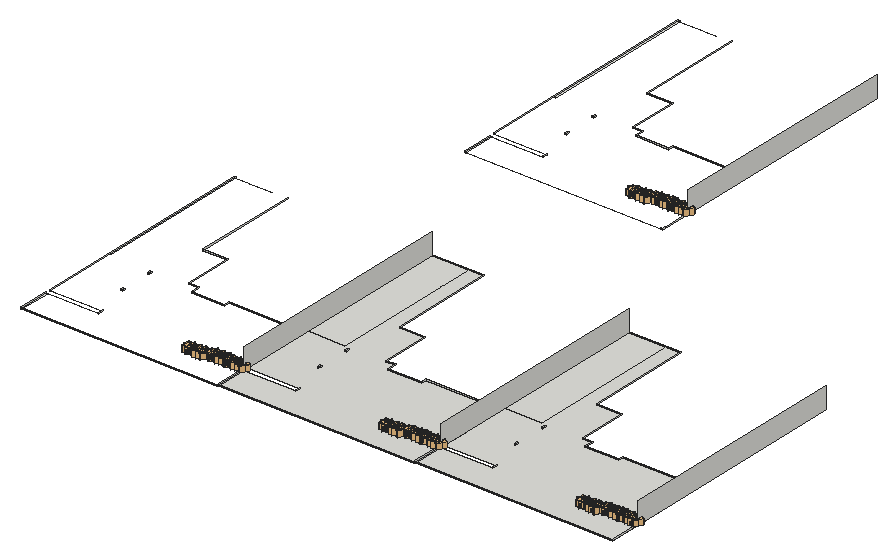
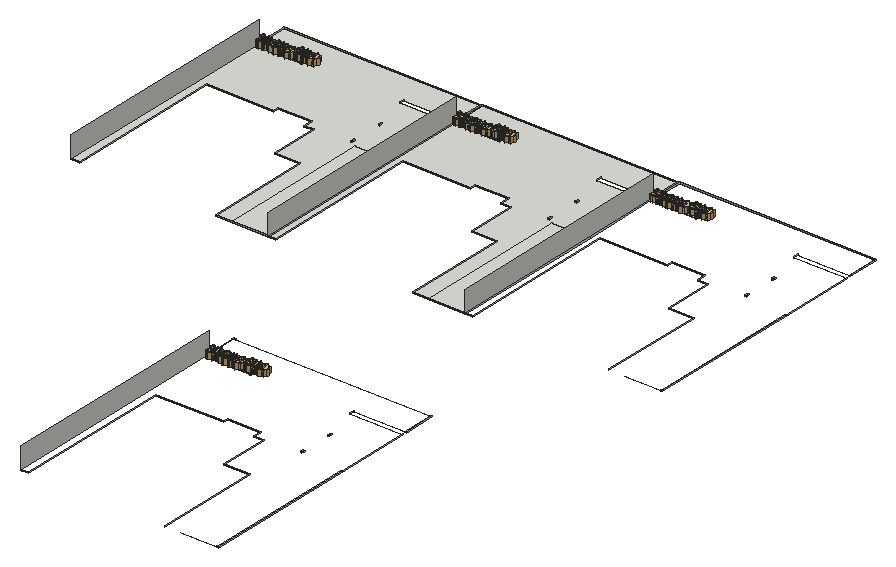
# SketchUp Ruby script. Lengths in inches.
U = 1.inch
M = Sketchup.active_model
def pt(a) = Geom::Point3d.new(a.map { |v| v * U })
def face(e, loops, mat)
  f = e.add_face(loops[0].map { |a| pt(a) })
  loops[1..].each { |l| e.add_face(l.map { |a| pt(a) }).erase! }
  f.material = f.back_material = mat if mat
  f
end
# faces: each face lists its corners as indices into pts; further lists are holes
def faces(e, pts, list, mat = nil) = list.each { |f| face(e, (f[0].is_a?(Array) ? f : [f]).map { |l| l.map { |i| pts[i] } }, mat) }
# xy, xz, yz: faces in a plane at the given z, y or x. An outline is a flat list of corners, or four numbers for a rectangle; further outlines are holes
def ring(l) = l.size == 4 ? [[l[0], l[1]], [l[2], l[1]], [l[2], l[3]], [l[0], l[3]]] : l.each_slice(2).to_a
def flat(e, list, mat, &to3) = list.each { |f| face(e, (f[0].is_a?(Array) ? f : [f]).map { |l| ring(l).map { |u, v| to3.(u, v) } }, mat) }
def xy(e, z, list, mat = nil) = flat(e, list, mat) { |x, y| [x, y, z] }
def xz(e, y, list, mat = nil) = flat(e, list, mat) { |x, z| [x, y, z] }
def yz(e, x, list, mat = nil) = flat(e, list, mat) { |y, z| [x, y, z] }
def lines(e, pts, list) = list.each { |a, b| e.add_line(pt(pts[a]), pt(pts[b])) }
# prism: a flat outline (further loops are holes) pulled along v
def prism(e, loops, v, mat = nil)
  f = face(e, loops, mat); d = Geom::Vector3d.new(v.map { |x| x * U })
  f.pushpull(f.normal.samedirection?(d) ? d.length : -d.length)
end
def box(e, o, s, mat = nil) = prism(e, [[o, [o[0] + s[0], o[1], o[2]], [o[0] + s[0], o[1] + s[1], o[2]], [o[0], o[1] + s[1], o[2]]]], [0, 0, s[2]], mat)
def at(x, y, z, deg = 0) = Geom::Transformation.translation(pt([x, y, z])) * Geom::Transformation.rotation(ORIGIN, Z_AXIS, deg.degrees)
def axes(o, x, y, z) = Geom::Transformation.new([*x, 0, *y, 0, *z, 0, *pt(o).to_a, 1])
def part(name) = M.definitions.add(name)
# library, detail: a bought-in or finely detailed component or shape, given as its bounding box
def library(name, o, s) = part(name).tap { |d| box(d.entities, o, s) }
def detail(e, o, s) = box(e.add_group.entities, o, s)
def put(e, d, t, mat = nil) = e.add_instance(d, t).tap { |i| i.material = mat if mat }
def group(e, t, mat = nil) = e.add_group.tap { |g| g.transformation = t; g.material = mat if mat }.entities
root = M.entities
M.materials.add("[Color_F16]").color = [51, 102, 0]
M.materials.add("[Field Square Tile]").color = [217, 201, 169]
c1 = library("Obj_000003",[-31,-31.06,-7.89],[62,62.12,39.58])
xy(root,-23.875,[[68.91,0,75.99,143.39],[955.37,0,962.46,143.39],[[962.46,0,962.46,143.39,1194.85,143.39,1194.85,164.82,962.46,164.82,962.46,505.3125,1127.79,505.3125,1127.79,1201.875,1196.48,1201.875,1196.48,726.125,1310.86,726.125,1310.86,505.3125,1354.48,505.3125,1354.48,464.0625,1504.89,464.0625,1504.89,487.3125,1810.23,487.3125,1810.23,1201.875,1841.83,1201.875,1841.83,164.82,1848.92,164.82,1848.92,143.39,1841.83,143.39,1841.83,0],[1150.61,475.3125,1157.34,487.3125],[1150.61,322.71,1157.34,334.4375]],[1841.83,0,1848.92,143.39],[[1848.92,0,1848.92,143.39,2081.32,143.39,2081.32,164.82,1848.92,164.82,1848.92,505.3125,2014.26,505.3125,2014.26,1201.875,2082.95,1201.875,2082.95,726.125,2197.32,726.125,2197.32,505.3125,2240.94,505.3125,2240.94,464.0625,2391.36,464.0625,2391.36,487.3125,2696.7,487.3125,2696.7,1201.875,2735.38,1201.875,2735.38,0],[2037.07,475.3125,2043.8,487.3125],[2037.07,322.71,2043.8,334.4375]],
  [955.37,164.82,962.46,505.3125],[1841.83,164.82,1848.92,505.3125],[68.91,505.3125,75.99,1201.875],[955.37,505.3125,962.46,1201.875],[962.46,505.3125,1127.79,1201.875],
  [1841.83,505.3125,1848.92,1201.875],[1848.92,505.3125,2014.26,1201.875],[587.64,1851.99,594.72,1995.38],[587.64,2357.31,594.72,3053.87]])
xy(root,-20.8125,[[747.55,143.39,901.18,164.82],[1634.02,143.39,1787.65,164.82],[2520.48,143.39,2674.11,164.82],[1266.28,1995.38,1419.92,2016.82]])
xz(root,0,[[75.99,-23.875,955.37,-19.3125],[955.37,-23.875,962.46,-19.3125],[962.46,-23.875,1841.83,-19.3125],[1841.83,-23.875,1848.92,-19.3125],[1848.92,-23.875,2735.38,-19.3125]],"[Field Square Tile]")
xz(root,143.39,[[747.55,-20.8125,901.18,-19.75],[1634.02,-20.8125,1787.65,-19.75],[2520.48,-20.8125,2674.11,-19.75]])
xz(root,164.82,[[747.55,-20.8125,901.18,-19.75],[1634.02,-20.8125,1787.65,-19.75],[2520.48,-20.8125,2674.11,-19.75]])
xz(root,322.71,[[264.14,-23.875,270.875,-19.75],[1150.61,-23.875,1157.34,-19.75],[2037.07,-23.875,2043.8,-19.75]])
xz(root,334.4375,[[264.14,-23.875,270.875,-19.75],[1150.61,-23.875,1157.34,-19.75],[2037.07,-23.875,2043.8,-19.75]])
xz(root,464.0625,[[468.02,-23.875,618.43,-19.75],[1354.48,-23.875,1504.89,-19.75],[2240.94,-23.875,2391.36,-19.75]])
xz(root,475.3125,[[264.14,-23.875,270.875,-19.75],[1150.61,-23.875,1157.34,-19.75],[2037.07,-23.875,2043.8,-19.75]])
xz(root,487.3125,[[264.14,-23.875,270.875,-19.75],[618.43,-23.875,923.77,-19.75],[1150.61,-23.875,1157.34,-19.75],[1504.89,-23.875,1810.23,-19.75],[2037.07,-23.875,2043.8,-19.75],
  [2391.36,-23.875,2696.7,-19.75]])
xz(root,505.3125,[[424.39,-23.875,468.02,-19.75],[1310.86,-23.875,1354.48,-19.75],[2197.32,-23.875,2240.94,-19.75]])
xz(root,726.125,[[310.02,-23.875,424.39,-19.75],[1196.48,-23.875,1310.86,-19.75],[2082.95,-23.875,2197.32,-19.75]])
xz(root,1201.875,[[68.91,-23.875,75.99,-19.75],[923.77,-23.875,955.37,-19.75],[955.37,-23.875,962.46,-19.75],[962.46,-23.875,1196.48,-19.75],[1810.23,-23.875,1841.83,-19.75],
  [1841.83,-23.875,1848.92,-19.75],[1848.92,-23.875,2082.95,-19.75],[2696.7,-23.875,2735.38,-19.75]])
xz(root,1851.99,[[1474.1,-23.875,1481.1875,-19.3125]],"[Field Square Tile]")
xz(root,1995.38,[[1266.28,-20.8125,1419.92,-19.75]])
xz(root,2016.82,[[1266.28,-20.8125,1419.92,-19.75]])
xz(root,2174.7,[[782.875,-23.875,789.61,-19.75]])
xz(root,2186.43,[[782.875,-23.875,789.61,-19.75]])
xz(root,2316.06,[[986.75,-23.875,1137.16,-19.75]])
xz(root,2327.31,[[782.875,-23.875,789.61,-19.75]])
xz(root,2339.31,[[782.875,-23.875,789.61,-19.75],[1137.16,-23.875,1442.5,-19.75]])
xz(root,2357.31,[[943.125,-23.875,986.75,-19.75]])
xz(root,2578.12,[[828.75,-23.875,943.125,-19.75]])
xz(root,3053.87,[[587.64,-23.875,594.72,-19.75],[1442.5,-23.875,1474.1,-19.75]])
yz(root,68.91,[[0,-23.875,0,-19.3125,12.39,-19.3125,12.39,-19.75,143.39,-19.75,143.39,-23.875],[164.82,-23.875,505.3125,-19.75],[505.3125,-23.875,1201.875,-19.75]])
yz(root,264.14,[[322.71,-23.875,334.4375,-19.75],[475.3125,-23.875,487.3125,-19.75]])
yz(root,270.875,[[322.71,-23.875,334.4375,-19.75],[475.3125,-23.875,487.3125,-19.75]])
yz(root,308.39,[[143.39,-23.875,164.82,-19.75]])
yz(root,310.02,[[726.125,-23.875,1201.875,-19.75]])
yz(root,424.39,[[505.3125,-23.875,726.125,-19.75]])
yz(root,468.02,[[464.0625,-23.875,505.3125,-19.75]])
yz(root,587.64,[[1851.99,-23.875,1851.99,-19.3125,1864.38,-19.3125,1864.38,-19.75,1995.38,-19.75,1995.38,-23.875],[2016.82,-23.875,2357.31,-19.75],[2357.31,-23.875,3053.87,-19.75]])
yz(root,618.43,[[464.0625,-23.875,487.3125,-19.75]])
yz(root,782.875,[[2174.7,-23.875,2186.43,-19.75],[2327.31,-23.875,2339.31,-19.75]])
yz(root,789.61,[[2174.7,-23.875,2186.43,-19.75],[2327.31,-23.875,2339.31,-19.75]])
yz(root,827.12,[[1995.38,-23.875,2016.82,-19.75]])
yz(root,828.75,[[2578.12,-23.875,3053.87,-19.75]])
yz(root,923.77,[[487.3125,-23.875,1201.875,-19.75]])
yz(root,943.125,[[2357.31,-23.875,2578.12,-19.75]])
yz(root,955.37,[[0,-23.875,0,-19.3125,12.39,-19.3125,12.39,-19.75,143.39,-19.75,143.39,-23.875],[164.82,-23.875,505.3125,-19.75],[505.3125,-23.875,1201.875,-19.75]])
yz(root,962.46,[[0,-23.875,1201.875,-23.875,1201.875,73,143.39,73,143.39,-19.75,12.39,-19.75,12.39,-19.3125,0,-19.3125]])
yz(root,986.75,[[2316.06,-23.875,2357.31,-19.75]])
yz(root,1137.16,[[2316.06,-23.875,2339.31,-19.75]])
yz(root,1150.61,[[322.71,-23.875,334.4375,-19.75],[475.3125,-23.875,487.3125,-19.75]])
yz(root,1157.34,[[322.71,-23.875,334.4375,-19.75],[475.3125,-23.875,487.3125,-19.75]])
yz(root,1194.85,[[143.39,-23.875,164.82,-19.75]])
yz(root,1196.48,[[726.125,-23.875,1201.875,-19.75]])
yz(root,1310.86,[[505.3125,-23.875,726.125,-19.75]])
yz(root,1354.48,[[464.0625,-23.875,505.3125,-19.75]])
yz(root,1442.5,[[2339.31,-23.875,3053.87,-19.75]])
yz(root,1481.1875,[[1851.99,-23.875,3053.87,-23.875,3053.87,73,1995.38,73,1995.38,-19.75,1864.38,-19.75,1864.38,-19.3125,1851.99,-19.3125]])
yz(root,1504.89,[[464.0625,-23.875,487.3125,-19.75]])
yz(root,1810.23,[[487.3125,-23.875,1201.875,-19.75]])
yz(root,1841.83,[[0,-23.875,0,-19.3125,12.39,-19.3125,12.39,-19.75,143.39,-19.75,143.39,-23.875],[164.82,-23.875,505.3125,-19.75],[505.3125,-23.875,1201.875,-19.75]])
yz(root,1848.92,[[0,-23.875,1201.875,-23.875,1201.875,73,143.39,73,143.39,-19.75,12.39,-19.75,12.39,-19.3125,0,-19.3125]])
yz(root,2037.07,[[322.71,-23.875,334.4375,-19.75],[475.3125,-23.875,487.3125,-19.75]])
yz(root,2043.8,[[322.71,-23.875,334.4375,-19.75],[475.3125,-23.875,487.3125,-19.75]])
yz(root,2081.32,[[143.39,-23.875,164.82,-19.75]])
yz(root,2082.95,[[726.125,-23.875,1201.875,-19.75]])
yz(root,2197.32,[[505.3125,-23.875,726.125,-19.75]])
yz(root,2240.94,[[464.0625,-23.875,505.3125,-19.75]])
yz(root,2391.36,[[464.0625,-23.875,487.3125,-19.75]])
yz(root,2696.7,[[487.3125,-23.875,1201.875,-19.75]])
yz(root,2735.38,[[0,-23.875,1201.875,-23.875,1201.875,73,143.39,73,143.39,-19.75,12.39,-19.75,12.39,-19.3125,0,-19.3125]])
p = [[308.39,164.82,-23.875],[75.99,164.82,-23.875],[241.33,1201.875,-23.875],[75.99,1201.875,-23.875],[75.99,143.39,-23.875],[308.39,143.39,-23.875],
  [68.91,164.82,-23.875],[594.72,1851.99,-19.3125],[594.72,1851.99,-23.875],[760.06,3053.87,-23.875],[594.72,3053.87,-23.875],[827.12,2016.82,-23.875],
  [594.72,2016.82,-23.875],[594.72,1995.38,-23.875],[827.12,1995.38,-23.875],[587.64,2016.82,-23.875],[1474.1,1851.99,-23.875]]
lines(root,p,[[0,1],[2,3],[4,5],[1,6],[7,8],[9,10],[11,12],[13,14],[12,15],[8,16]])
put(root,c1,axes([1630.48,130.4,-17.02],[-0.16941,0.61717,-0.00035],[-0.61717,-0.16941,0.00015],[0.00005,0.00038,0.64]),"[Color_F16]")
put(root,c1,axes([1662.26,130.18,-17.02],[0.45255,0.45255,-0.00035],[-0.45255,0.45255,0.00015],[0.00035,0.00015,0.64]),"[Color_F16]")
put(root,c1,axes([1646.38,130.18,-17.02],[0.45255,0.45255,-0.00035],[-0.45255,0.45255,0.00015],[0.00035,0.00015,0.64]),"[Color_F16]")
put(root,c1,axes([1614.64,130.18,-17.02],[0.45255,0.45255,-0.00035],[-0.45255,0.45255,0.00015],[0.00035,0.00015,0.64]),"[Color_F16]")
put(root,c1,axes([1676.95,129.48,-17.02],[0.34155,0.54124,-0.00035],[-0.54124,0.34155,0.00015],[0.00031,0.00022,0.64]),"[Color_F16]")
put(root,c1,axes([2501.1,130.18,-17.02],[0.45255,0.45255,-0.00035],[-0.45255,0.45255,0.00015],[0.00035,0.00015,0.64]),"[Color_F16]")
put(root,c1,axes([2563.41,129.48,-17.02],[0.34155,0.54124,-0.00035],[-0.54124,0.34155,0.00015],[0.00031,0.00022,0.64]),"[Color_F16]")
put(root,c1,axes([2516.95,130.4,-17.02],[-0.16941,0.61717,-0.00035],[-0.61717,-0.16941,0.00015],[0.00005,0.00038,0.64]),"[Color_F16]")
put(root,c1,axes([2548.72,130.18,-17.02],[0.45255,0.45255,-0.00035],[-0.45255,0.45255,0.00015],[0.00035,0.00015,0.64]),"[Color_F16]")
put(root,c1,axes([2532.85,130.18,-17.02],[0.45255,0.45255,-0.00035],[-0.45255,0.45255,0.00015],[0.00035,0.00015,0.64]),"[Color_F16]")
put(root,c1,axes([790.48,129.48,-17.02],[0.34155,0.54124,-0.00035],[-0.54124,0.34155,0.00015],[0.00031,0.00022,0.64]),"[Color_F16]")
put(root,c1,axes([744.02,130.4,-17.02],[-0.16941,0.61717,-0.00035],[-0.61717,-0.16941,0.00015],[0.00005,0.00038,0.64]),"[Color_F16]")
put(root,c1,axes([728.17,130.18,-17.02],[0.45255,0.45255,-0.00035],[-0.45255,0.45255,0.00015],[0.00035,0.00015,0.64]),"[Color_F16]")
put(root,c1,axes([775.79,130.18,-17.02],[0.45255,0.45255,-0.00035],[-0.45255,0.45255,0.00015],[0.00035,0.00015,0.64]),"[Color_F16]")
put(root,c1,axes([759.92,130.18,-17.02],[0.45255,0.45255,-0.00035],[-0.45255,0.45255,0.00015],[0.00035,0.00015,0.64]),"[Color_F16]")
put(root,c1,axes([1278.65,1982.18,-17.02],[0.45255,0.45255,-0.00035],[-0.45255,0.45255,0.00015],[0.00035,0.00015,0.64]),"[Color_F16]")
put(root,c1,axes([1294.53,1982.18,-17.02],[0.45255,0.45255,-0.00035],[-0.45255,0.45255,0.00015],[0.00035,0.00015,0.64]),"[Color_F16]")
put(root,c1,axes([1262.75,1982.39,-17.02],[-0.16941,0.61717,-0.00035],[-0.61717,-0.16941,0.00015],[0.00005,0.00038,0.64]),"[Color_F16]")
put(root,c1,axes([1246.9,1982.18,-17.02],[0.45255,0.45255,-0.00035],[-0.45255,0.45255,0.00015],[0.00035,0.00015,0.64]),"[Color_F16]")
put(root,c1,axes([1309.22,1981.47,-17.02],[0.34155,0.54124,-0.00035],[-0.54124,0.34155,0.00015],[0.00031,0.00022,0.64]),"[Color_F16]")
put(root,c1,axes([1677.44,130.52,-17.02],[0.28256,0.57425,0],[-0.57425,0.28256,0],[0,0,0.64]),"[Color_F16]")
put(root,c1,axes([1614.23,130.26,-17.02],[0.64,0,0],[0,0.64,0],[0,0,0.64]),"[Color_F16]")
put(root,c1,axes([1630.48,130.71,-17.02],[-0.15049,0.62206,0],[-0.62206,-0.15049,0],[0,0,0.64]),"[Color_F16]")
put(root,c1,axes([1645.97,130.26,-17.02],[0.64,0,0],[0,0.64,0],[0,0,0.64]),"[Color_F16]")
put(root,c1,axes([1661.85,130.26,-17.02],[0.64,0,0],[0,0.64,0],[0,0,0.64]),"[Color_F16]")
put(root,c1,axes([2532.4375,130.26,-17.02],[0.64,0,0],[0,0.64,0],[0,0,0.64]),"[Color_F16]")
put(root,c1,axes([2563.9,130.52,-17.02],[0.28256,0.57425,0],[-0.57425,0.28256,0],[0,0,0.64]),"[Color_F16]")
put(root,c1,axes([2500.69,130.26,-17.02],[0.64,0,0],[0,0.64,0],[0,0,0.64]),"[Color_F16]")
put(root,c1,axes([2516.95,130.71,-17.02],[-0.15049,0.62206,0],[-0.62206,-0.15049,0],[0,0,0.64]),"[Color_F16]")
put(root,c1,axes([2548.3125,130.26,-17.02],[0.64,0,0],[0,0.64,0],[0,0,0.64]),"[Color_F16]")
put(root,c1,axes([759.51,130.26,-17.02],[0.64,0,0],[0,0.64,0],[0,0,0.64]),"[Color_F16]")
put(root,c1,axes([727.76,130.26,-17.02],[0.64,0,0],[0,0.64,0],[0,0,0.64]),"[Color_F16]")
put(root,c1,axes([790.97,130.52,-17.02],[0.28256,0.57425,0],[-0.57425,0.28256,0],[0,0,0.64]),"[Color_F16]")
put(root,c1,axes([744.02,130.71,-17.02],[-0.15049,0.62206,0],[-0.62206,-0.15049,0],[0,0,0.64]),"[Color_F16]")
put(root,c1,axes([775.38,130.26,-17.02],[0.64,0,0],[0,0.64,0],[0,0,0.64]),"[Color_F16]")
put(root,c1,axes([1262.75,1982.71,-17.02],[-0.15049,0.62206,0],[-0.62206,-0.15049,0],[0,0,0.64]),"[Color_F16]")
put(root,c1,axes([1309.7,1982.52,-17.02],[0.28256,0.57425,0],[-0.57425,0.28256,0],[0,0,0.64]),"[Color_F16]")
put(root,c1,axes([1278.24,1982.25,-17.02],[0.64,0,0],[0,0.64,0],[0,0,0.64]),"[Color_F16]")
put(root,c1,axes([1246.49,1982.25,-17.02],[0.64,0,0],[0,0.64,0],[0,0,0.64]),"[Color_F16]")
put(root,c1,axes([1294.12,1982.25,-17.02],[0.64,0,0],[0,0.64,0],[0,0,0.64]),"[Color_F16]")
put(root,c1,axes([1708.47,144.13,-16.22],[0.45255,0.45255,-0.00035],[-0.45255,0.45255,0.00015],[0.00035,0.00015,0.64]),"[Color_F16]")
put(root,c1,axes([1770.79,143.43,-16.22],[0.34155,0.54124,-0.00035],[-0.54124,0.34155,0.00015],[0.00031,0.00022,0.64]),"[Color_F16]")
put(root,c1,axes([1724.32,144.35,-16.22],[-0.16941,0.61717,-0.00035],[-0.61717,-0.16941,0.00015],[0.00005,0.00038,0.64]),"[Color_F16]")
put(root,c1,axes([1756.1,144.13,-16.22],[0.45255,0.45255,-0.00035],[-0.45255,0.45255,0.00015],[0.00035,0.00015,0.64]),"[Color_F16]")
put(root,c1,axes([1740.22,144.13,-16.22],[0.45255,0.45255,-0.00035],[-0.45255,0.45255,0.00015],[0.00035,0.00015,0.64]),"[Color_F16]")
put(root,c1,axes([1841.16,143.43,-16.22],[0.34155,0.54124,-0.00035],[-0.54124,0.34155,0.00015],[0.00031,0.00022,0.64]),"[Color_F16]")
put(root,c1,axes([1778.85,144.13,-16.22],[0.45255,0.45255,-0.00035],[-0.45255,0.45255,0.00015],[0.00035,0.00015,0.64]),"[Color_F16]")
put(root,c1,axes([1794.7,144.35,-16.22],[-0.16941,0.61717,-0.00035],[-0.61717,-0.16941,0.00015],[0.00005,0.00038,0.64]),"[Color_F16]")
put(root,c1,axes([1826.47,144.13,-16.22],[0.45255,0.45255,-0.00035],[-0.45255,0.45255,0.00015],[0.00035,0.00015,0.64]),"[Color_F16]")
put(root,c1,axes([1810.6,144.13,-16.22],[0.45255,0.45255,-0.00035],[-0.45255,0.45255,0.00015],[0.00035,0.00015,0.64]),"[Color_F16]")
put(root,c1,axes([2697.06,144.13,-16.22],[0.45255,0.45255,-0.00035],[-0.45255,0.45255,0.00015],[0.00035,0.00015,0.64]),"[Color_F16]")
put(root,c1,axes([2712.93,144.13,-16.22],[0.45255,0.45255,-0.00035],[-0.45255,0.45255,0.00015],[0.00035,0.00015,0.64]),"[Color_F16]")
put(root,c1,axes([2681.16,144.35,-16.22],[-0.16941,0.61717,-0.00035],[-0.61717,-0.16941,0.00015],[0.00005,0.00038,0.64]),"[Color_F16]")
put(root,c1,axes([2665.3125,144.13,-16.22],[0.45255,0.45255,-0.00035],[-0.45255,0.45255,0.00015],[0.00035,0.00015,0.64]),"[Color_F16]")
put(root,c1,axes([2727.625,143.43,-16.22],[0.34155,0.54124,-0.00035],[-0.54124,0.34155,0.00015],[0.00031,0.00022,0.64]),"[Color_F16]")
put(root,c1,axes([2657.25,143.43,-16.22],[0.34155,0.54124,-0.00035],[-0.54124,0.34155,0.00015],[0.00031,0.00022,0.64]),"[Color_F16]")
put(root,c1,axes([2594.9375,144.13,-16.22],[0.45255,0.45255,-0.00035],[-0.45255,0.45255,0.00015],[0.00035,0.00015,0.64]),"[Color_F16]")
put(root,c1,axes([2610.79,144.35,-16.22],[-0.16941,0.61717,-0.00035],[-0.61717,-0.16941,0.00015],[0.00005,0.00038,0.64]),"[Color_F16]")
put(root,c1,axes([2642.56,144.13,-16.22],[0.45255,0.45255,-0.00035],[-0.45255,0.45255,0.00015],[0.00035,0.00015,0.64]),"[Color_F16]")
put(root,c1,axes([2626.69,144.13,-16.22],[0.45255,0.45255,-0.00035],[-0.45255,0.45255,0.00015],[0.00035,0.00015,0.64]),"[Color_F16]")
put(root,c1,axes([892.38,144.13,-16.22],[0.45255,0.45255,-0.00035],[-0.45255,0.45255,0.00015],[0.00035,0.00015,0.64]),"[Color_F16]")
put(root,c1,axes([908.23,144.35,-16.22],[-0.16941,0.61717,-0.00035],[-0.61717,-0.16941,0.00015],[0.00005,0.00038,0.64]),"[Color_F16]")
put(root,c1,axes([924.13,144.13,-16.22],[0.45255,0.45255,-0.00035],[-0.45255,0.45255,0.00015],[0.00035,0.00015,0.64]),"[Color_F16]")
put(root,c1,axes([940.01,144.13,-16.22],[0.45255,0.45255,-0.00035],[-0.45255,0.45255,0.00015],[0.00035,0.00015,0.64]),"[Color_F16]")
put(root,c1,axes([954.7,143.43,-16.22],[0.34155,0.54124,-0.00035],[-0.54124,0.34155,0.00015],[0.00031,0.00022,0.64]),"[Color_F16]")
put(root,c1,axes([884.32,143.43,-16.22],[0.34155,0.54124,-0.00035],[-0.54124,0.34155,0.00015],[0.00031,0.00022,0.64]),"[Color_F16]")
put(root,c1,axes([822.01,144.13,-16.22],[0.45255,0.45255,-0.00035],[-0.45255,0.45255,0.00015],[0.00035,0.00015,0.64]),"[Color_F16]")
put(root,c1,axes([869.63,144.13,-16.22],[0.45255,0.45255,-0.00035],[-0.45255,0.45255,0.00015],[0.00035,0.00015,0.64]),"[Color_F16]")
put(root,c1,axes([837.86,144.35,-16.22],[-0.16941,0.61717,-0.00035],[-0.61717,-0.16941,0.00015],[0.00005,0.00038,0.64]),"[Color_F16]")
put(root,c1,axes([853.76,144.13,-16.22],[0.45255,0.45255,-0.00035],[-0.45255,0.45255,0.00015],[0.00035,0.00015,0.64]),"[Color_F16]")
put(root,c1,axes([1442.86,1996.125,-16.22],[0.45255,0.45255,-0.00035],[-0.45255,0.45255,0.00015],[0.00035,0.00015,0.64]),"[Color_F16]")
put(root,c1,axes([1403.05,1995.42,-16.22],[0.34155,0.54124,-0.00035],[-0.54124,0.34155,0.00015],[0.00031,0.00022,0.64]),"[Color_F16]")
put(root,c1,axes([1340.74,1996.125,-16.22],[0.45255,0.45255,-0.00035],[-0.45255,0.45255,0.00015],[0.00035,0.00015,0.64]),"[Color_F16]")
put(root,c1,axes([1388.36,1996.125,-16.22],[0.45255,0.45255,-0.00035],[-0.45255,0.45255,0.00015],[0.00035,0.00015,0.64]),"[Color_F16]")
put(root,c1,axes([1458.74,1996.125,-16.22],[0.45255,0.45255,-0.00035],[-0.45255,0.45255,0.00015],[0.00035,0.00015,0.64]),"[Color_F16]")
put(root,c1,axes([1411.12,1996.125,-16.22],[0.45255,0.45255,-0.00035],[-0.45255,0.45255,0.00015],[0.00035,0.00015,0.64]),"[Color_F16]")
put(root,c1,axes([1426.96,1996.34,-16.22],[-0.16941,0.61717,-0.00035],[-0.61717,-0.16941,0.00015],[0.00005,0.00038,0.64]),"[Color_F16]")
put(root,c1,axes([1473.43,1995.42,-16.22],[0.34155,0.54124,-0.00035],[-0.54124,0.34155,0.00015],[0.00031,0.00022,0.64]),"[Color_F16]")
put(root,c1,axes([1356.59,1996.34,-16.22],[-0.16941,0.61717,-0.00035],[-0.61717,-0.16941,0.00015],[0.00005,0.00038,0.64]),"[Color_F16]")
put(root,c1,axes([1372.49,1996.125,-16.22],[0.45255,0.45255,-0.00035],[-0.45255,0.45255,0.00015],[0.00035,0.00015,0.64]),"[Color_F16]")
put(root,c1,axes([1739.8125,144.21,-16.22],[0.64,0,0],[0,0.64,0],[0,0,0.64]),"[Color_F16]")
put(root,c1,axes([1771.27,144.47,-16.22],[0.28256,0.57425,0],[-0.57425,0.28256,0],[0,0,0.64]),"[Color_F16]")
put(root,c1,axes([1708.0625,144.21,-16.22],[0.64,0,0],[0,0.64,0],[0,0,0.64]),"[Color_F16]")
put(root,c1,axes([1724.32,144.66,-16.22],[-0.15049,0.62206,0],[-0.62206,-0.15049,0],[0,0,0.64]),"[Color_F16]")
put(root,c1,axes([1755.6875,144.21,-16.22],[0.64,0,0],[0,0.64,0],[0,0,0.64]),"[Color_F16]")
put(root,c1,axes([1778.4375,144.21,-16.22],[0.64,0,0],[0,0.64,0],[0,0,0.64]),"[Color_F16]")
put(root,c1,axes([1841.65,144.47,-16.22],[0.28256,0.57425,0],[-0.57425,0.28256,0],[0,0,0.64]),"[Color_F16]")
put(root,c1,axes([1810.1875,144.21,-16.22],[0.64,0,0],[0,0.64,0],[0,0,0.64]),"[Color_F16]")
put(root,c1,axes([1794.7,144.66,-16.22],[-0.15049,0.62206,0],[-0.62206,-0.15049,0],[0,0,0.64]),"[Color_F16]")
put(root,c1,axes([1826.0625,144.21,-16.22],[0.64,0,0],[0,0.64,0],[0,0,0.64]),"[Color_F16]")
put(root,c1,axes([2728.11,144.47,-16.22],[0.28256,0.57425,0],[-0.57425,0.28256,0],[0,0,0.64]),"[Color_F16]")
put(root,c1,axes([2664.9,144.21,-16.22],[0.64,0,0],[0,0.64,0],[0,0,0.64]),"[Color_F16]")
put(root,c1,axes([2681.16,144.66,-16.22],[-0.15049,0.62206,0],[-0.62206,-0.15049,0],[0,0,0.64]),"[Color_F16]")
put(root,c1,axes([2712.52,144.21,-16.22],[0.64,0,0],[0,0.64,0],[0,0,0.64]),"[Color_F16]")
put(root,c1,axes([2696.65,144.21,-16.22],[0.64,0,0],[0,0.64,0],[0,0,0.64]),"[Color_F16]")
put(root,c1,axes([2594.53,144.21,-16.22],[0.64,0,0],[0,0.64,0],[0,0,0.64]),"[Color_F16]")
put(root,c1,axes([2657.74,144.47,-16.22],[0.28256,0.57425,0],[-0.57425,0.28256,0],[0,0,0.64]),"[Color_F16]")
put(root,c1,axes([2626.28,144.21,-16.22],[0.64,0,0],[0,0.64,0],[0,0,0.64]),"[Color_F16]")
put(root,c1,axes([2610.79,144.66,-16.22],[-0.15049,0.62206,0],[-0.62206,-0.15049,0],[0,0,0.64]),"[Color_F16]")
put(root,c1,axes([2642.15,144.21,-16.22],[0.64,0,0],[0,0.64,0],[0,0,0.64]),"[Color_F16]")
put(root,c1,axes([939.6,144.21,-16.22],[0.64,0,0],[0,0.64,0],[0,0,0.64]),"[Color_F16]")
put(root,c1,axes([955.18,144.47,-16.22],[0.28256,0.57425,0],[-0.57425,0.28256,0],[0,0,0.64]),"[Color_F16]")
put(root,c1,axes([891.97,144.21,-16.22],[0.64,0,0],[0,0.64,0],[0,0,0.64]),"[Color_F16]")
put(root,c1,axes([908.23,144.66,-16.22],[-0.15049,0.62206,0],[-0.62206,-0.15049,0],[0,0,0.64]),"[Color_F16]")
put(root,c1,axes([923.72,144.21,-16.22],[0.64,0,0],[0,0.64,0],[0,0,0.64]),"[Color_F16]")
put(root,c1,axes([884.81,144.47,-16.22],[0.28256,0.57425,0],[-0.57425,0.28256,0],[0,0,0.64]),"[Color_F16]")
put(root,c1,axes([821.6,144.21,-16.22],[0.64,0,0],[0,0.64,0],[0,0,0.64]),"[Color_F16]")
put(root,c1,axes([869.22,144.21,-16.22],[0.64,0,0],[0,0.64,0],[0,0,0.64]),"[Color_F16]")
put(root,c1,axes([837.86,144.66,-16.22],[-0.15049,0.62206,0],[-0.62206,-0.15049,0],[0,0,0.64]),"[Color_F16]")
put(root,c1,axes([853.35,144.21,-16.22],[0.64,0,0],[0,0.64,0],[0,0,0.64]),"[Color_F16]")
put(root,c1,axes([1403.54,1996.47,-16.22],[0.28256,0.57425,0],[-0.57425,0.28256,0],[0,0,0.64]),"[Color_F16]")
put(root,c1,axes([1473.92,1996.47,-16.22],[0.28256,0.57425,0],[-0.57425,0.28256,0],[0,0,0.64]),"[Color_F16]")
put(root,c1,axes([1458.33,1996.2,-16.22],[0.64,0,0],[0,0.64,0],[0,0,0.64]),"[Color_F16]")
put(root,c1,axes([1442.45,1996.2,-16.22],[0.64,0,0],[0,0.64,0],[0,0,0.64]),"[Color_F16]")
put(root,c1,axes([1387.95,1996.2,-16.22],[0.64,0,0],[0,0.64,0],[0,0,0.64]),"[Color_F16]")
put(root,c1,axes([1340.33,1996.2,-16.22],[0.64,0,0],[0,0.64,0],[0,0,0.64]),"[Color_F16]")
put(root,c1,axes([1356.59,1996.66,-16.22],[-0.15049,0.62206,0],[-0.62206,-0.15049,0],[0,0,0.64]),"[Color_F16]")
put(root,c1,axes([1410.71,1996.2,-16.22],[0.64,0,0],[0,0.64,0],[0,0,0.64]),"[Color_F16]")
put(root,c1,axes([1426.96,1996.66,-16.22],[-0.15049,0.62206,0],[-0.62206,-0.15049,0],[0,0,0.64]),"[Color_F16]")
put(root,c1,axes([1372.08,1996.2,-16.22],[0.64,0,0],[0,0.64,0],[0,0,0.64]),"[Color_F16]")
